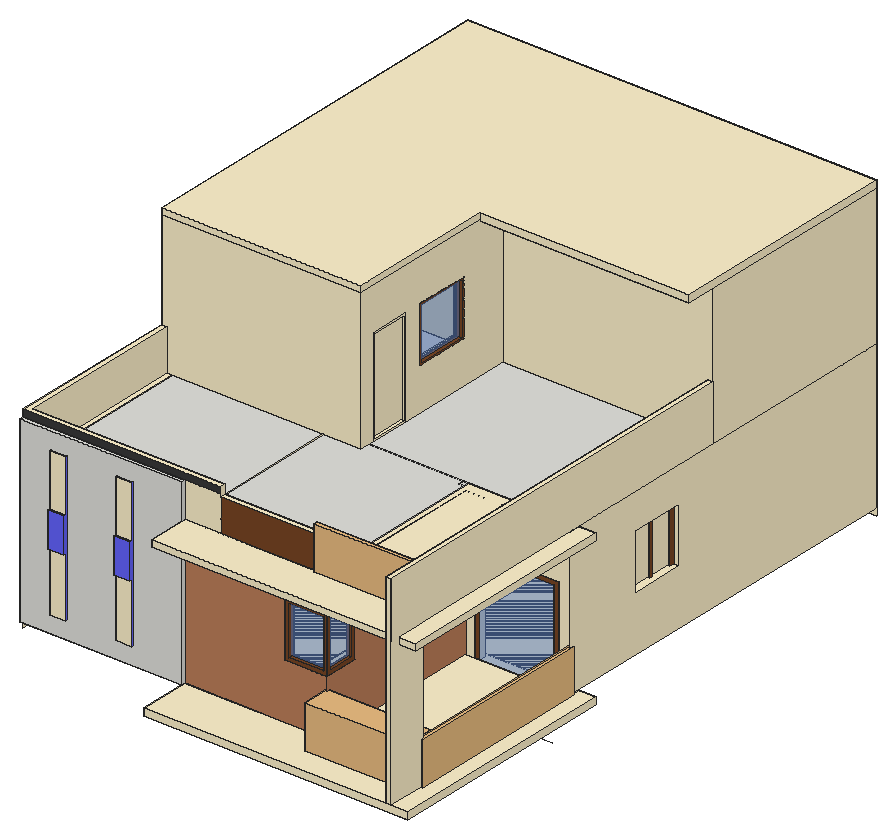
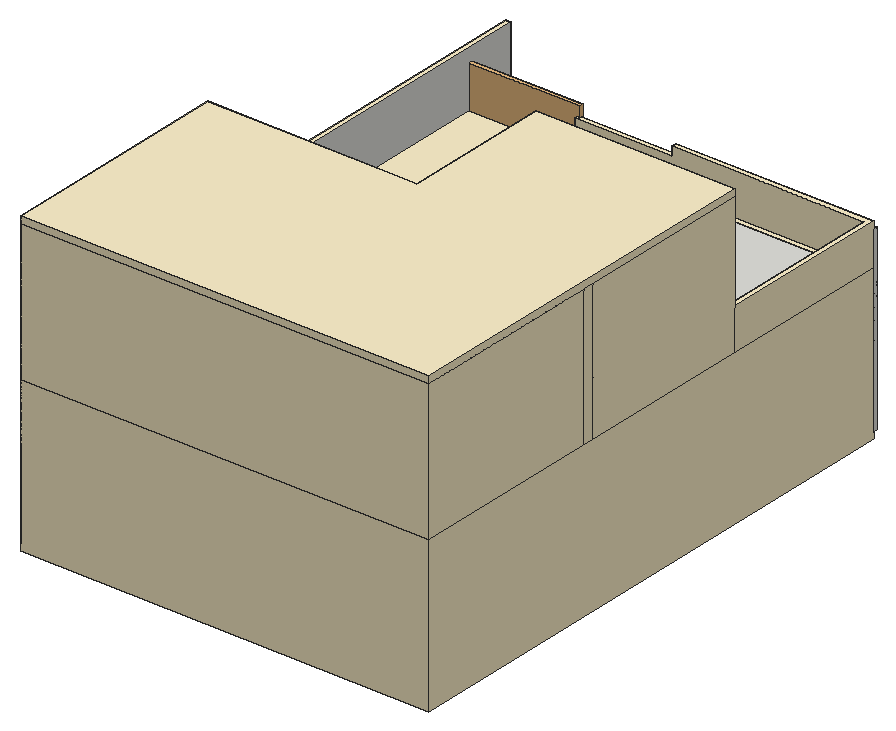
# SketchUp Ruby script. Lengths in inches.
U = 1.inch
M = Sketchup.active_model
def pt(a) = Geom::Point3d.new(a.map { |v| v * U })
def face(e, loops, mat)
  f = e.add_face(loops[0].map { |a| pt(a) })
  loops[1..].each { |l| e.add_face(l.map { |a| pt(a) }).erase! }
  f.material = f.back_material = mat if mat
  f
end
# faces: each face lists its corners as indices into pts; further lists are holes
def faces(e, pts, list, mat = nil) = list.each { |f| face(e, (f[0].is_a?(Array) ? f : [f]).map { |l| l.map { |i| pts[i] } }, mat) }
# xy, xz, yz: faces in a plane at the given z, y or x. An outline is a flat list of corners, or four numbers for a rectangle; further outlines are holes
def ring(l) = l.size == 4 ? [[l[0], l[1]], [l[2], l[1]], [l[2], l[3]], [l[0], l[3]]] : l.each_slice(2).to_a
def flat(e, list, mat, &to3) = list.each { |f| face(e, (f[0].is_a?(Array) ? f : [f]).map { |l| ring(l).map { |u, v| to3.(u, v) } }, mat) }
def xy(e, z, list, mat = nil) = flat(e, list, mat) { |x, y| [x, y, z] }
def xz(e, y, list, mat = nil) = flat(e, list, mat) { |x, z| [x, y, z] }
def yz(e, x, list, mat = nil) = flat(e, list, mat) { |y, z| [x, y, z] }
def lines(e, pts, list) = list.each { |a, b| e.add_line(pt(pts[a]), pt(pts[b])) }
# prism: a flat outline (further loops are holes) pulled along v
def prism(e, loops, v, mat = nil)
  f = face(e, loops, mat); d = Geom::Vector3d.new(v.map { |x| x * U })
  f.pushpull(f.normal.samedirection?(d) ? d.length : -d.length)
end
def box(e, o, s, mat = nil) = prism(e, [[o, [o[0] + s[0], o[1], o[2]], [o[0] + s[0], o[1] + s[1], o[2]], [o[0], o[1] + s[1], o[2]]]], [0, 0, s[2]], mat)
def at(x, y, z, deg = 0) = Geom::Transformation.translation(pt([x, y, z])) * Geom::Transformation.rotation(ORIGIN, Z_AXIS, deg.degrees)
def axes(o, x, y, z) = Geom::Transformation.new([*x, 0, *y, 0, *z, 0, *pt(o).to_a, 1])
def part(name) = M.definitions.add(name)
# library, detail: a bought-in or finely detailed component or shape, given as its bounding box
def library(name, o, s) = part(name).tap { |d| box(d.entities, o, s) }
def detail(e, o, s) = box(e.add_group.entities, o, s)
def put(e, d, t, mat = nil) = e.add_instance(d, t).tap { |i| i.material = mat if mat }
def group(e, t, mat = nil) = e.add_group.tap { |g| g.transformation = t; g.material = mat if mat }.entities
root = M.entities
M.materials.add("[Color D01]").color = [255, 242, 204]
M.materials.add("[Color I03]").color = [101, 101, 255]
M.materials.add("[Color M07]").color = [58, 58, 58]
M.materials.add("[Translucent Glass Blue]").color = [100, 149, 237]
M.materials["[Translucent Glass Blue]"].alpha = 0.5
M.materials.add("[Wood Cherry Original]").color = [152, 86, 42]
M.materials.add("[Wood Veneer 01]").color = [120, 70, 37]
M.materials.add("[Wood Veneer 02]").color = [190, 128, 91]
c1 = part("Group99\#2")
xy(c1.entities,0,[[0,0,19,44]])
c2 = part("Group97\#1")
xy(c2.entities,0,[[0,0,0,48,48,48,48,0,44,0,44,44,25,44,25,0,23,0,23,44,4,44,4,0]])
xy(c2.entities,4,[[0,0,4,0,4,44,23,44,23,0,25,0,25,44,44,44,44,0,48,0,48,48,0,48]],"[Wood Veneer 01]")
xz(c2.entities,0,[[0,0,4,4],[23,0,25,4],[44,0,48,4]])
xz(c2.entities,44,[[4,0,23,4],[25,0,44,4]])
xz(c2.entities,48,[[0,0,48,4]])
yz(c2.entities,0,[[0,0,48,4]])
yz(c2.entities,4,[[0,0,44,4]])
yz(c2.entities,23,[[0,0,44,4]])
yz(c2.entities,25,[[0,0,44,4]])
yz(c2.entities,44,[[0,0,44,4]])
yz(c2.entities,48,[[0,0,48,4]])
p = [[23,0,0],[4,0,0],[44,0,0],[25,0,0],[0.08,0.08,0],[0.08,0.08,4]]
lines(c2.entities,p,[[0,1],[2,3],[4,5]])
put(c2.entities,c1,at(4,0,2))
put(c2.entities,c1,at(25,0,2))
c3 = part("Group103\#1")
xy(c3.entities,0,[[-36,-42,-36,42,36,42,36,-42,32,-42,32,38,-32,38,-32,-42]])
xy(c3.entities,5.875,[[-36,-42,-32,-42,-32,38,32,38,32,-42,36,-42,36,42,-36,42]],"[Wood Veneer 01]")
xz(c3.entities,-42,[[-36,0,-32,5.875],[32,0,36,5.875]])
xz(c3.entities,38,[[-32,0,32,5.875]])
xz(c3.entities,42,[[-36,0,36,5.875]])
yz(c3.entities,-36,[[-42,0,42,5.875]])
yz(c3.entities,-32,[[-42,0,38,5.875]])
yz(c3.entities,32,[[-42,0,38,5.875]])
yz(c3.entities,36,[[-42,0,42,5.875]])
c4 = part("Difference")
xy(c4.entities,0,[[9,9,256.5,9,256.5,153,252,153,252,157.5,269.25,157.5,269.25,148.5,341.25,148.5,341.25,157.5,342,157.5,342,468,9,468]])
xy(c4.entities,48,[[225,0,261,0,261,30,256.5,30,256.5,9,225,9],[342,217.5,351,265.5]])
xy(c4.entities,84,[[269.25,148.5,341.25,157.5]])
xy(c4.entities,96,[[225,0,225,9,256.5,9,256.5,30,261,30,261,0],[342,217.5,351,265.5]])
xy(c4.entities,125.875,[[[0,0,261,0,261,148.5,351,148.5,351,477,0,477],[9,9,9,468,342,468,342,157.5,252,157.5,252,153,256.5,153,256.5,9]]])
xz(c4.entities,0,[[0,0,138.625,125.875]])
xz(c4.entities,0,[[138.625,0,261,0,261,48,225,48,225,96,261,96,261,125.875,138.625,125.875]],"[Wood Veneer 02]")
xz(c4.entities,9,[[9,0,9,125.875,256.5,125.875,256.5,96,225,96,225,48,256.5,48,256.5,0]])
xz(c4.entities,30,[[256.5,48,261,96]])
xz(c4.entities,148.5,[[261,-6,269.25,-6,269.25,84,341.25,84,341.25,-6,351,-6,351,125.875,261,125.875],[269.25,-6,341.25,0]])
xz(c4.entities,153,[[252,-6,256.5,0],[252,0,256.5,125.875]])
xz(c4.entities,157.5,[[252,-6,269.25,0],[341.25,-6,342,0],[252,0,252,125.875,342,125.875,342,0,341.25,0,341.25,84,269.25,84,269.25,0]])
xz(c4.entities,217.5,[[342,48,351,96]])
xz(c4.entities,265.5,[[342,48,351,96]])
xz(c4.entities,468,[[9,-6,342,0],[9,0,342,125.875]])
xz(c4.entities,477,[[0,-6,351,125.875]])
yz(c4.entities,0,[[0,-6,477,125.875]])
yz(c4.entities,9,[[9,0,468,125.875]])
yz(c4.entities,225,[[0,48,9,96]])
yz(c4.entities,252,[[153,-6,157.5,0],[153,0,157.5,125.875]])
yz(c4.entities,256.5,[[9,0,9,48,30,48,30,96,9,96,9,125.875,153,125.875,153,0]])
yz(c4.entities,261,[[0,0,148.5,0,148.5,125.875,0,125.875,0,96,30,96,30,48,0,48]],"[Wood Veneer 02]")
yz(c4.entities,269.25,[[148.5,-6,157.5,0],[148.5,0,157.5,84]])
yz(c4.entities,341.25,[[148.5,-6,157.5,0],[148.5,0,157.5,84]])
yz(c4.entities,342,[[157.5,-6,468,0],[[157.5,0,468,125.875],[217.5,48,265.5,96]]])
yz(c4.entities,351,[[[148.5,0,477,125.875],[217.5,48,265.5,96]]])
p = [[261,0,-6],[261,0,0],[9,9,0],[9,9,-6],[261,0,96],[261,0,48],
  [256.5,9,0],[256.5,9,-6],[138.625,0,125.875],[138.625,0,126]]
lines(c4.entities,p,[[0,1],[2,3],[4,5],[6,7],[8,9]])
put(c4.entities,c2,axes([342,217.5,48],[0,1,0],[0,0,1],[1,0,0]))
put(c4.entities,c3,axes([305.25,154.375,42],[1,0,0],[0,0,1],[0,-1,0]))
c5 = library("Group\#8",[0,0,0],[89.04,23.58,36.98])
c6 = library("Group\#9",[0,0,0],[3.15,162.6875,36.98])
c7 = part("Group92\#1")
p = [[33,3,0],[3,3,0],[3,45,0],[33,45,0]]
lines(c7.entities,p,[[0,1],[1,2],[2,3],[3,0]])
c8 = part("Group93\#1")
xy(c8.entities,2.5,[[3,3,33,45]])
c9 = part("Group91\#1")
xy(c9.entities,5,[[[0,0,36,48],[3,3,33,45]]],"[Wood Veneer 01]")
xz(c9.entities,0,[[0,0,36,5]],"[Wood Veneer 01]")
xz(c9.entities,3,[[3,0,33,5]],"[Wood Veneer 01]")
xz(c9.entities,45,[[3,0,33,5]],"[Wood Veneer 01]")
xz(c9.entities,48,[[0,0,36,5]],"[Wood Veneer 01]")
yz(c9.entities,0,[[0,0,48,5]],"[Wood Veneer 01]")
yz(c9.entities,3,[[3,0,45,5]],"[Wood Veneer 01]")
yz(c9.entities,33,[[3,0,45,5]],"[Wood Veneer 01]")
put(c9.entities,c7,at(0,0,0))
put(c9.entities,c8,at(0,0,0),"[Translucent Glass Blue]")
c10 = part("Group95\#1")
p = [[3,-45,0],[3,-3,0],[27,-3,0],[27,-45,0]]
lines(c10.entities,p,[[0,1],[1,2],[2,3],[3,0]])
c11 = part("Group96\#1")
xy(c11.entities,2.5,[[3,-45,27,-3]])
c12 = part("Group94\#1")
xy(c12.entities,5,[[[0,-48,30,0],[3,-45,27,-3]]],"[Wood Veneer 01]")
xz(c12.entities,-48,[[0,0,30,5]],"[Wood Veneer 01]")
xz(c12.entities,-45,[[3,0,27,5]],"[Wood Veneer 01]")
xz(c12.entities,-3,[[3,0,27,5]],"[Wood Veneer 01]")
xz(c12.entities,0,[[0,0,30,5]],"[Wood Veneer 01]")
yz(c12.entities,3,[[-45,0,-3,5]],"[Wood Veneer 01]")
yz(c12.entities,27,[[-45,0,-3,5]],"[Wood Veneer 01]")
yz(c12.entities,30,[[-48,0,0,5]],"[Wood Veneer 01]")
put(c12.entities,c10,at(0,0,0))
put(c12.entities,c11,at(0,0,0),"[Translucent Glass Blue]")
c13 = part("Group120\#1")
p = [[46.8125,1.1875,0],[1.1875,1.1875,0],[1.1875,46.68,0],[46.8125,46.68,0]]
lines(c13.entities,p,[[0,1],[1,2],[2,3],[3,0]])
c14 = part("Group121\#1")
xy(c14.entities,2.9375,[[1.1875,1.1875,46.8125,46.68]],"[Translucent Glass Blue]")
c15 = part("Group119\#1")
xy(c15.entities,0,[[[0,0,48,47.87],[1.1875,1.1875,46.8125,46.68]]])
xy(c15.entities,5.875,[[[0,0,48,47.87],[1.1875,1.1875,46.8125,46.68]]],"[Wood Veneer 01]")
xz(c15.entities,0,[[0,0,48,5.875]])
xz(c15.entities,1.1875,[[1.1875,0,46.8125,5.875]],"[Wood Veneer 01]")
xz(c15.entities,46.68,[[1.1875,0,46.8125,5.875]])
xz(c15.entities,47.87,[[0,0,48,5.875]])
yz(c15.entities,0,[[0,0,47.87,5.875]])
yz(c15.entities,1.1875,[[1.1875,0,46.68,5.875]])
yz(c15.entities,46.8125,[[1.1875,0,46.68,5.875]],"[Wood Veneer 01]")
yz(c15.entities,48,[[0,0,47.87,5.875]])
put(c15.entities,c13,at(0,0,0))
put(c15.entities,c14,at(0,0,0))
c16 = part("Group117\#1")
p = [[-1.1875,82.8125,0],[-1.1875,1.1875,0],[-34.8125,1.1875,0],[-34.8125,82.8125,0]]
lines(c16.entities,p,[[0,1],[1,2],[2,3],[3,0]])
c17 = part("Group118\#1")
xy(c17.entities,2.9375,[[-34.8125,1.1875,-1.1875,82.8125]])
c18 = part("Group116\#1")
prism(c18.entities,[[[-36,84,0],[0,84,0],[0,0,0],[-36,0,0]],[[-1.1875,1.1875,0],[-1.1875,82.8125,0],[-34.8125,82.8125,0],[-34.8125,1.1875,0]]],[0,0,5.875])
put(c18.entities,c16,at(0,0,0))
put(c18.entities,c17,at(0,0,0))
c19 = library("Group\#10",[0,0,0],[97.38,3.15,36.98])
xy(root,136,[[388.5,16.4375,393,49.75],[42,57,180.625,60]])
xy(root,151.2,[[68.16,55.5,82.23,57],[124.79,55.5,138.85,57]])
xy(root,202.6,[[68.16,53.5,82.23,55.5],[124.79,53.5,138.85,55.5]])
xy(root,232.56,[[68.16,53.5,82.23,55.5],[124.79,53.5,138.85,55.5]])
xy(root,277.2,[[68.16,55.5,82.23,57],[124.79,55.5,138.85,57]])
xy(root,292.05,[[42,57,180.625,60]])
xz(root,16.4375,[[388.5,136,393,310]],"[Color D01]")
xz(root,49.75,[[388.5,136,393,262]],"[Color D01]")
xz(root,53.5,[[68.16,202.6,82.23,232.56],[124.79,202.6,138.85,232.56]],"[Color I03]")
xz(root,55.5,[[68.16,151.2,82.23,202.6],[124.79,151.2,138.85,202.6],[68.16,232.56,82.23,277.2],[124.79,232.56,138.85,277.2]],"[Color D01]")
xz(root,57,[[[42,136,180.625,292.05],[68.16,151.2,82.23,277.2],[124.79,151.2,138.85,277.2]]])
xz(root,60,[[42,136,180.625,292.05]])
yz(root,42,[[57,136,60,292.05]])
yz(root,68.16,[[55.5,151.2,55.5,202.6,53.5,202.6,53.5,232.56,55.5,232.56,55.5,277.2,57,277.2,57,151.2]])
yz(root,82.23,[[55.5,151.2,57,151.2,57,277.2,55.5,277.2,55.5,232.56,53.5,232.56,53.5,202.6,55.5,202.6]],"[Color I03]")
yz(root,124.79,[[55.5,151.2,55.5,202.6,53.5,202.6,53.5,232.56,55.5,232.56,55.5,277.2,57,277.2,57,151.2]])
yz(root,138.85,[[55.5,151.2,57,151.2,57,277.2,55.5,277.2,55.5,232.56,53.5,232.56,53.5,202.6,55.5,202.6]],"[Color I03]")
yz(root,180.625,[[57,136,60,292.05]])
yz(root,388.5,[[16.4375,262,361.5,310]])
yz(root,388.5,[[16.4375,136,49.75,262]],"[Color D01]")
yz(root,393,[[16.4375,136,49.75,136,49.75,262,361.5,262,361.5,310,16.4375,310]],"[Color D01]")
p = [[303,60,184],[303,90,184],[378,208.5,94],[330,208.5,94]]
lines(root,p,[[0,1],[2,3]])
put(root,c4,at(42,60,136),"[Color D01]")
g1 = group(root,at(51,45,130),"[Color D01]")
prism(g1,[[[21,168,0],[21,172.5,0],[0,172.5,0],[0,316.5,0],[0,321,0],[0,483,0],[132,483,0],[136.5,483,0],[190.5,483,0],[195,483,0],[333,483,0],[333,172.5,0],[186,172.5,0],[186,24,0],[21,24,0]]],[0,0,6])
prism(g1,[[[357,172.5,0],[357,-29.1,0],[129.625,-29.1,0],[129.625,15,0],[195,15,0],[195,163.5,0],[342,163.5,0],[342,172.5,0]]],[0,0,6])
g2 = group(root,at(315.25,208.5,136))
xz(g2,0,[[0,0,64,80]],"[Translucent Glass Blue]")
put(root,c5,at(301.43,38.38,136))
put(root,c6,at(391.43,47.78,136))
put(root,c9,axes([267,65,184],[1,0,0],[0,0,1],[0,-1,0]))
put(root,c12,axes([298,60,232],[0,1,0],[0,0,1],[1,0,0]))
g3 = group(root,at(237,45,256),"[Color D01]")
xy(g3,0,[[[-56.375,-20.6,171,172.5],[105.02,-5.04,106.57,-4.84,108.02,-4.24,109.26,-3.28,110.21,-2.04,110.8125,-0.59,111.02,0.96,110.8125,2.51,110.21,3.96,109.26,5.2,108.02,6.16,106.57,6.76,105.02,6.96,103.46,6.76,102.02,6.16,100.77,5.2,99.82,3.96,99.22,2.51,99.02,0.96,99.22,-0.59,99.82,-2.04,100.77,-3.28,102.02,-4.24,103.46,-4.84],[29.7,-5.04,31.26,-4.84,32.7,-4.24,33.95,-3.28,34.9,-2.04,35.5,-0.59,35.7,0.96,35.5,2.51,34.9,3.96,33.95,5.2,32.7,6.16,31.26,6.76,29.7,6.96,28.15,6.76,26.7,6.16,25.46,5.2,24.51,3.96,23.91,2.51,23.7,0.96,23.91,-0.59,24.51,-2.04,25.46,-3.28,26.7,-4.24,28.15,-4.84],[-29.86,-5.04,-28.31,-4.84,-26.86,-4.24,-25.62,-3.28,-24.66,-2.04,-24.0625,-0.59,-23.86,0.96,-24.0625,2.51,-24.66,3.96,-25.62,5.2,-26.86,6.16,-28.31,6.76,-29.86,6.96,-31.41,6.76,-32.86,6.16,-34.1,5.2,-35.05,3.96,-35.65,2.51,-35.86,0.96,-35.65,-0.59,-35.05,-2.04,-34.1,-3.28,-32.86,-4.24,-31.41,-4.84],[147.08,-5.04,148.63,-4.84,150.08,-4.24,151.32,-3.28,152.28,-2.04,152.875,-0.59,153.08,0.96,152.875,2.51,152.28,3.96,151.32,5.2,150.08,6.16,148.63,6.76,147.08,6.96,145.53,6.76,144.08,6.16,142.84,5.2,141.88,3.96,141.28,2.51,141.08,0.96,141.28,-0.59,141.88,-2.04,142.84,-3.28,144.08,-4.24,145.53,-4.84],[91.35,86.46,92.9,86.66,94.35,87.26,95.59,88.22,96.54,89.46,97.14,90.91,97.35,92.46,97.14,94.01,96.54,95.46,95.59,96.7,94.35,97.66,92.9,98.26,91.35,98.46,89.79,98.26,88.35,97.66,87.1,96.7,86.15,95.46,85.55,94.01,85.35,92.46,85.55,90.91,86.15,89.46,87.1,88.22,88.35,87.26,89.79,86.66],[149.66,86.46,151.21,86.66,152.66,87.26,153.9,88.22,154.85,89.46,155.45,90.91,155.66,92.46,155.45,94.01,154.85,95.46,153.9,96.7,152.66,97.66,151.21,98.26,149.66,98.46,148.11,98.26,146.66,97.66,145.42,96.7,144.46,95.46,143.86,94.01,143.66,92.46,143.86,90.91,144.46,89.46,145.42,88.22,146.66,87.26,148.11,86.66]]],"[Wood Cherry Original]")
xy(g3,1,[[-29.86,-5.04,-31.41,-4.84,-32.86,-4.24,-34.1,-3.28,-35.05,-2.04,-35.65,-0.59,-35.86,0.96,-35.65,2.51,-35.05,3.96,-34.1,5.2,-32.86,6.16,-31.41,6.76,-29.86,6.96,-28.31,6.76,-26.86,6.16,-25.62,5.2,-24.66,3.96,-24.0625,2.51,-23.86,0.96,-24.0625,-0.59,-24.66,-2.04,-25.62,-3.28,-26.86,-4.24,-28.31,-4.84],[29.7,-5.04,28.15,-4.84,26.7,-4.24,25.46,-3.28,24.51,-2.04,23.91,-0.59,23.7,0.96,23.91,2.51,24.51,3.96,25.46,5.2,26.7,6.16,28.15,6.76,29.7,6.96,31.26,6.76,32.7,6.16,33.95,5.2,34.9,3.96,35.5,2.51,35.7,0.96,35.5,-0.59,34.9,-2.04,33.95,-3.28,32.7,-4.24,31.26,-4.84],[105.02,-5.04,103.46,-4.84,102.02,-4.24,100.77,-3.28,99.82,-2.04,99.22,-0.59,99.02,0.96,99.22,2.51,99.82,3.96,100.77,5.2,102.02,6.16,103.46,6.76,105.02,6.96,106.57,6.76,108.02,6.16,109.26,5.2,110.21,3.96,110.8125,2.51,111.02,0.96,110.8125,-0.59,110.21,-2.04,109.26,-3.28,108.02,-4.24,106.57,-4.84],[147.08,-5.04,145.53,-4.84,144.08,-4.24,142.84,-3.28,141.88,-2.04,141.28,-0.59,141.08,0.96,141.28,2.51,141.88,3.96,142.84,5.2,144.08,6.16,145.53,6.76,147.08,6.96,148.63,6.76,150.08,6.16,151.32,5.2,152.28,3.96,152.875,2.51,153.08,0.96,152.875,-0.59,152.28,-2.04,151.32,-3.28,150.08,-4.24,148.63,-4.84],[91.35,86.46,89.79,86.66,88.35,87.26,87.1,88.22,86.15,89.46,85.55,90.91,85.35,92.46,85.55,94.01,86.15,95.46,87.1,96.7,88.35,97.66,89.79,98.26,91.35,98.46,92.9,98.26,94.35,97.66,95.59,96.7,96.54,95.46,97.14,94.01,97.35,92.46,97.14,90.91,96.54,89.46,95.59,88.22,94.35,87.26,92.9,86.66],
  [149.66,86.46,148.11,86.66,146.66,87.26,145.42,88.22,144.46,89.46,143.86,90.91,143.66,92.46,143.86,94.01,144.46,95.46,145.42,96.7,146.66,97.66,148.11,98.26,149.66,98.46,151.21,98.26,152.66,97.66,153.9,96.7,154.85,95.46,155.45,94.01,155.66,92.46,155.45,90.91,154.85,89.46,153.9,88.22,152.66,87.26,151.21,86.66]])
xy(g3,6,[[-56.375,-20.6,171,172.5]])
xz(g3,-20.6,[[-56.375,0,171,6]])
xz(g3,172.5,[[-56.375,0,171,6]])
yz(g3,-56.375,[[-20.6,0,172.5,6]])
yz(g3,171,[[-20.6,0,172.5,6]])
p = [[-29.86,-5.04,0],[-31.41,-4.84,0],[-31.41,-4.84,1],[-29.86,-5.04,1],[-28.31,-4.84,0],[-28.31,-4.84,1],
  [29.7,-5.04,0],[28.15,-4.84,0],[28.15,-4.84,1],[29.7,-5.04,1],[31.26,-4.84,0],[31.26,-4.84,1],
  [105.02,-5.04,0],[103.46,-4.84,0],[103.46,-4.84,1],[105.02,-5.04,1],[106.57,-4.84,0],[106.57,-4.84,1],
  [147.08,-5.04,0],[145.53,-4.84,0],[145.53,-4.84,1],[147.08,-5.04,1],[148.63,-4.84,0],[148.63,-4.84,1],
  [-32.86,-4.24,0],[-32.86,-4.24,1],[-26.86,-4.24,0],[-26.86,-4.24,1],[26.7,-4.24,0],[26.7,-4.24,1],
  [32.7,-4.24,0],[32.7,-4.24,1],[102.02,-4.24,0],[102.02,-4.24,1],[108.02,-4.24,0],[108.02,-4.24,1],
  [144.08,-4.24,0],[144.08,-4.24,1],[150.08,-4.24,0],[150.08,-4.24,1],[-34.1,-3.28,0],[-34.1,-3.28,1],
  [-25.62,-3.28,0],[-25.62,-3.28,1],[25.46,-3.28,0],[25.46,-3.28,1],[33.95,-3.28,0],[33.95,-3.28,1],
  [100.77,-3.28,0],[100.77,-3.28,1],[109.26,-3.28,0],[109.26,-3.28,1],[142.84,-3.28,0],[142.84,-3.28,1],
  [151.32,-3.28,0],[151.32,-3.28,1],[-35.05,-2.04,0],[-35.05,-2.04,1],[-24.66,-2.04,0],[-24.66,-2.04,1],
  [24.51,-2.04,0],[24.51,-2.04,1],[34.9,-2.04,0],[34.9,-2.04,1],[99.82,-2.04,0],[99.82,-2.04,1],
  [110.21,-2.04,0],[110.21,-2.04,1],[141.88,-2.04,0],[141.88,-2.04,1],[152.28,-2.04,0],[152.28,-2.04,1],
  [-35.65,-0.59,0],[-35.65,-0.59,1],[-24.0625,-0.59,0],[-24.0625,-0.59,1],[23.91,-0.59,0],[23.91,-0.59,1],
  [35.5,-0.59,0],[35.5,-0.59,1],[99.22,-0.59,0],[99.22,-0.59,1],[110.8125,-0.59,0],[110.8125,-0.59,1],
  [141.28,-0.59,0],[141.28,-0.59,1],[152.875,-0.59,0],[152.875,-0.59,1],[-35.86,0.96,0],[-35.86,0.96,1],
  [-23.86,0.96,0],[-23.86,0.96,1],[23.7,0.96,0],[23.7,0.96,1],[35.7,0.96,0],[35.7,0.96,1],
  [99.02,0.96,0],[99.02,0.96,1],[111.02,0.96,0],[111.02,0.96,1],[141.08,0.96,0],[141.08,0.96,1],
  [153.08,0.96,0],[153.08,0.96,1],[-35.65,2.51,0],[-35.65,2.51,1],[-24.0625,2.51,0],[-24.0625,2.51,1],
  [23.91,2.51,0],[23.91,2.51,1],[35.5,2.51,0],[35.5,2.51,1],[99.22,2.51,0],[99.22,2.51,1],
  [110.8125,2.51,0],[110.8125,2.51,1],[141.28,2.51,0],[141.28,2.51,1],[152.875,2.51,0],[152.875,2.51,1],
  [-35.05,3.96,0],[-35.05,3.96,1],[-24.66,3.96,0],[-24.66,3.96,1],[24.51,3.96,0],[24.51,3.96,1],
  [34.9,3.96,0],[34.9,3.96,1],[99.82,3.96,0],[99.82,3.96,1],[110.21,3.96,0],[110.21,3.96,1],
  [141.88,3.96,0],[141.88,3.96,1],[152.28,3.96,0],[152.28,3.96,1],[-34.1,5.2,0],[-34.1,5.2,1],
  [-25.62,5.2,0],[-25.62,5.2,1],[25.46,5.2,0],[25.46,5.2,1],[33.95,5.2,0],[33.95,5.2,1],
  [100.77,5.2,0],[100.77,5.2,1],[109.26,5.2,0],[109.26,5.2,1],[142.84,5.2,0],[142.84,5.2,1],
  [151.32,5.2,0],[151.32,5.2,1],[-32.86,6.16,0],[-32.86,6.16,1],[-26.86,6.16,0],[-26.86,6.16,1],
  [26.7,6.16,0],[26.7,6.16,1],[32.7,6.16,0],[32.7,6.16,1],[102.02,6.16,0],[102.02,6.16,1],
  [108.02,6.16,0],[108.02,6.16,1],[144.08,6.16,0],[144.08,6.16,1],[150.08,6.16,0],[150.08,6.16,1],
  [-31.41,6.76,0],[-31.41,6.76,1],[-28.31,6.76,0],[-28.31,6.76,1],[28.15,6.76,0],[28.15,6.76,1],
  [31.26,6.76,0],[31.26,6.76,1],[103.46,6.76,0],[103.46,6.76,1],[106.57,6.76,0],[106.57,6.76,1],
  [145.53,6.76,0],[145.53,6.76,1],[148.63,6.76,0],[148.63,6.76,1],[-29.86,6.96,0],[-29.86,6.96,1],
  [29.7,6.96,0],[29.7,6.96,1],[105.02,6.96,0],[105.02,6.96,1],[147.08,6.96,0],[147.08,6.96,1],
  [91.35,86.46,0],[89.79,86.66,0],[89.79,86.66,1],[91.35,86.46,1],[92.9,86.66,0],[92.9,86.66,1],
  [149.66,86.46,0],[148.11,86.66,0],[148.11,86.66,1],[149.66,86.46,1],[151.21,86.66,0],[151.21,86.66,1],
  [88.35,87.26,0],[88.35,87.26,1],[94.35,87.26,0],[94.35,87.26,1],[146.66,87.26,0],[146.66,87.26,1],
  [152.66,87.26,0],[152.66,87.26,1],[87.1,88.22,0],[87.1,88.22,1],[95.59,88.22,0],[95.59,88.22,1],
  [145.42,88.22,0],[145.42,88.22,1],[153.9,88.22,0],[153.9,88.22,1],[86.15,89.46,0],[86.15,89.46,1],
  [96.54,89.46,0],[96.54,89.46,1],[144.46,89.46,0],[144.46,89.46,1],[154.85,89.46,0],[154.85,89.46,1],
  [85.55,90.91,0],[85.55,90.91,1],[97.14,90.91,0],[97.14,90.91,1],[143.86,90.91,0],[143.86,90.91,1],
  [155.45,90.91,0],[155.45,90.91,1],[85.35,92.46,0],[85.35,92.46,1],[97.35,92.46,0],[97.35,92.46,1],
  [143.66,92.46,0],[143.66,92.46,1],[155.66,92.46,0],[155.66,92.46,1],[85.55,94.01,0],[85.55,94.01,1],
  [97.14,94.01,0],[97.14,94.01,1],[143.86,94.01,0],[143.86,94.01,1],[155.45,94.01,0],[155.45,94.01,1],
  [86.15,95.46,0],[86.15,95.46,1],[96.54,95.46,0],[96.54,95.46,1],[144.46,95.46,0],[144.46,95.46,1],
  [154.85,95.46,0],[154.85,95.46,1],[87.1,96.7,0],[87.1,96.7,1],[95.59,96.7,0],[95.59,96.7,1],
  [145.42,96.7,0],[145.42,96.7,1],[153.9,96.7,0],[153.9,96.7,1],[88.35,97.66,0],[88.35,97.66,1],
  [94.35,97.66,0],[94.35,97.66,1],[146.66,97.66,0],[146.66,97.66,1],[152.66,97.66,0],[152.66,97.66,1],
  [89.79,98.26,0],[89.79,98.26,1],[92.9,98.26,0],[92.9,98.26,1],[148.11,98.26,0],[148.11,98.26,1],
  [151.21,98.26,0],[151.21,98.26,1],[91.35,98.46,0],[91.35,98.46,1],[149.66,98.46,0],[149.66,98.46,1]]
faces(g3,p,[[0,1,2,3],[4,0,3,5],[6,7,8,9],[10,6,9,11],[12,13,14,15],[16,12,15,17],[18,19,20,21],[22,18,21,23],
  [1,24,25,2],[26,4,5,27],[7,28,29,8],[30,10,11,31],[13,32,33,14],[34,16,17,35],[19,36,37,20],[38,22,23,39],
  [24,40,41,25],[42,26,27,43],[28,44,45,29],[46,30,31,47],[32,48,49,33],[50,34,35,51],[36,52,53,37],[54,38,39,55],
  [40,56,57,41],[58,42,43,59],[44,60,61,45],[62,46,47,63],[48,64,65,49],[66,50,51,67],[52,68,69,53],[70,54,55,71],
  [56,72,73,57],[74,58,59,75],[60,76,77,61],[78,62,63,79],[64,80,81,65],[82,66,67,83],[68,84,85,69],[86,70,71,87],
  [72,88,89,73],[90,74,75,91],[76,92,93,77],[94,78,79,95],[80,96,97,81],[98,82,83,99],[84,100,101,85],[102,86,87,103],
  [88,104,105,89],[106,90,91,107],[92,108,109,93],[110,94,95,111],[96,112,113,97],[114,98,99,115],[100,116,117,101],[118,102,103,119],
  [104,120,121,105],[122,106,107,123],[108,124,125,109],[126,110,111,127],[112,128,129,113],[130,114,115,131],[116,132,133,117],[134,118,119,135],
  [120,136,137,121],[138,122,123,139],[124,140,141,125],[142,126,127,143],[128,144,145,129],[146,130,131,147],[132,148,149,133],[150,134,135,151],
  [136,152,153,137],[154,138,139,155],[140,156,157,141],[158,142,143,159],[144,160,161,145],[162,146,147,163],[148,164,165,149],[166,150,151,167],
  [152,168,169,153],[170,154,155,171],[156,172,173,157],[174,158,159,175],[160,176,177,161],[178,162,163,179],[164,180,181,165],[182,166,167,183],
  [168,184,185,169],[184,170,171,185],[172,186,187,173],[186,174,175,187],[176,188,189,177],[188,178,179,189],[180,190,191,181],[190,182,183,191],
  [192,193,194,195],[196,192,195,197],[198,199,200,201],[202,198,201,203],[193,204,205,194],[206,196,197,207],[199,208,209,200],[210,202,203,211],
  [204,212,213,205],[214,206,207,215],[208,216,217,209],[218,210,211,219],[212,220,221,213],[222,214,215,223],[216,224,225,217],[226,218,219,227],
  [220,228,229,221],[230,222,223,231],[224,232,233,225],[234,226,227,235],[228,236,237,229],[238,230,231,239],[232,240,241,233],[242,234,235,243],
  [236,244,245,237],[246,238,239,247],[240,248,249,241],[250,242,243,251],[244,252,253,245],[254,246,247,255],[248,256,257,249],[258,250,251,259],
  [252,260,261,253],[262,254,255,263],[256,264,265,257],[266,258,259,267],[260,268,269,261],[270,262,263,271],[264,272,273,265],[274,266,267,275],
  [268,276,277,269],[278,270,271,279],[272,280,281,273],[282,274,275,283],[276,284,285,277],[284,278,279,285],[280,286,287,281],[286,282,283,287]])
g4 = group(root,at(-709.92,-151.5625,146.75))
prism(g4,[[[1008.42,369.0625,109.25],[1008.42,220.5625,109.25],[760.92,220.5625,109.25],[760.92,679.5625,109.25],[1093.92,679.5625,109.25],[1093.92,369.0625,109.25]]],[0,0,6])
g5 = group(root,at(42,60,262),"[Color D01]")
xy(g5,0,[[0,148.5,0,301.5,9,301.5,9,157.5,162,157.5,162,161.2,171,161.2,171,148.5],[162,161.2,171,197.2],[162,197.2,171,301.5],[[0,301.5,351,477],[9,310.5,342,468]]])
xy(g5,28.25,[[169.53,0,253.06,4.5]])
xy(g5,36,[[0,0,169.53,0,169.53,4.5,4.5,4.5,4.5,148.5,0,148.5]])
xy(g5,36.13,[[162,211.45,171,259.45]])
xy(g5,48,[[346.5,-43.5625,351,301.5]])
xy(g5,84,[[162,161.2,171,197.2]])
xy(g5,84.13,[[162,211.45,171,259.45]])
xy(g5,120,[[[0,148.5,171,148.5,171,301.5,351,301.5,351,477,0,477],[9,310.5,342,468],[9,157.5,162,301.5]]])
xz(g5,0,[[0,0,169.53,30.05]])
xz(g5,0,[[0,30.05,169.53,36]],"[Color M07]")
xz(g5,0,[[169.53,0,253.06,28.25]],"[Wood Veneer 01]")
xz(g5,4.5,[[169.53,-0.125,169.53,0,4.5,0,4.5,36,169.53,36,169.53,28.25,253.06,28.25,253.06,-0.125]])
xz(g5,148.5,[[0,0,4.5,36],[4.5,0,171,0,171,120,0,120,0,36,4.5,36]])
xz(g5,157.5,[[9,0,162,120]])
xz(g5,161.2,[[162,0,171,84]])
xz(g5,197.2,[[162,0,171,84]])
xz(g5,211.45,[[162,36.13,171,84],[162,84,171,84.13]])
xz(g5,259.45,[[162,36.13,171,84.13]])
xz(g5,301.5,[[9,0,162,120],[171,0,346.5,0,346.5,48,351,48,351,120,171,120],[346.5,0,351,48]])
xz(g5,310.5,[[9,0,342,120]])
xz(g5,468,[[9,0,342,120]])
xz(g5,477,[[0,0,351,120]])
yz(g5,0,[[0,0,148.5,36],[148.5,0,301.5,120],[301.5,0,310.5,120],[310.5,0,477,120]])
yz(g5,4.5,[[4.5,0,148.5,36]])
yz(g5,9,[[157.5,0,301.5,120],[310.5,0,468,120]])
yz(g5,162,[[[157.5,0,157.5,120,301.5,120,301.5,0,197.2,0,197.2,84,161.2,84,161.2,0],[211.45,36.13,259.45,84.13]]])
yz(g5,169.53,[[0,28.25,4.5,36]])
yz(g5,171,[[[148.5,0,161.2,0,161.2,84,197.2,84,197.2,0,301.5,0,301.5,120,148.5,120],[211.45,36.13,259.45,84.13]],[211.45,84,259.45,84.13]])
yz(g5,253.06,[[0,-0.125,4.5,28.25]])
yz(g5,342,[[310.5,0,468,120]])
yz(g5,351,[[301.5,0,477,120]])
p = [[102,262.5,0],[102,301.5,0],[351,-43.5625,0],[351,-43.5625,48],[346.5,-43.5625,0],[346.5,-43.5625,48]]
lines(g5,p,[[0,1],[2,3],[4,5]])
put(g5,c15,axes([165.125,211.45,36.13],[0,1,0],[0,0,1],[1,0,0]))
put(g5,c18,axes([165.125,197.2,0],[0,1,0],[0,0,1],[1,0,0]))
put(root,c19,at(293.09,58.43,262))
g6 = group(root,at(42,208.5,382),"[Color D01]")
prism(g6,[[[0,328.5,0],[351,328.5,0],[351,127.5625,0],[171,127.5625,0],[171,0,0],[0,0,0]]],[0,0,6])
